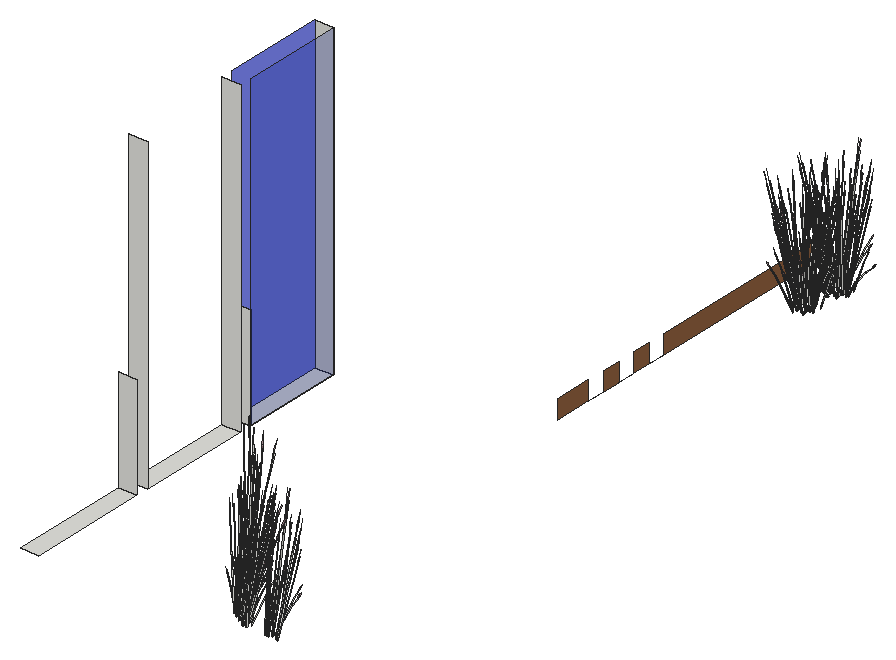
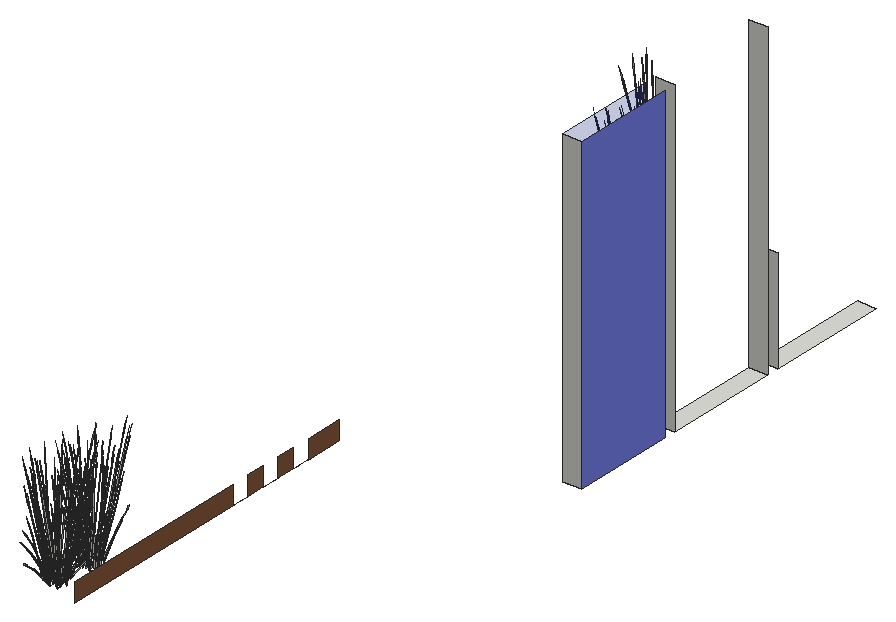
# SketchUp Ruby script. Lengths in inches.
U = 1.inch
M = Sketchup.active_model
def pt(a) = Geom::Point3d.new(a.map { |v| v * U })
def face(e, loops, mat)
  f = e.add_face(loops[0].map { |a| pt(a) })
  loops[1..].each { |l| e.add_face(l.map { |a| pt(a) }).erase! }
  f.material = f.back_material = mat if mat
  f
end
# faces: each face lists its corners as indices into pts; further lists are holes
def faces(e, pts, list, mat = nil) = list.each { |f| face(e, (f[0].is_a?(Array) ? f : [f]).map { |l| l.map { |i| pts[i] } }, mat) }
# xy, xz, yz: faces in a plane at the given z, y or x. An outline is a flat list of corners, or four numbers for a rectangle; further outlines are holes
def ring(l) = l.size == 4 ? [[l[0], l[1]], [l[2], l[1]], [l[2], l[3]], [l[0], l[3]]] : l.each_slice(2).to_a
def flat(e, list, mat, &to3) = list.each { |f| face(e, (f[0].is_a?(Array) ? f : [f]).map { |l| ring(l).map { |u, v| to3.(u, v) } }, mat) }
def xy(e, z, list, mat = nil) = flat(e, list, mat) { |x, y| [x, y, z] }
def xz(e, y, list, mat = nil) = flat(e, list, mat) { |x, z| [x, y, z] }
def yz(e, x, list, mat = nil) = flat(e, list, mat) { |y, z| [x, y, z] }
def lines(e, pts, list) = list.each { |a, b| e.add_line(pt(pts[a]), pt(pts[b])) }
# prism: a flat outline (further loops are holes) pulled along v
def prism(e, loops, v, mat = nil)
  f = face(e, loops, mat); d = Geom::Vector3d.new(v.map { |x| x * U })
  f.pushpull(f.normal.samedirection?(d) ? d.length : -d.length)
end
def box(e, o, s, mat = nil) = prism(e, [[o, [o[0] + s[0], o[1], o[2]], [o[0] + s[0], o[1] + s[1], o[2]], [o[0], o[1] + s[1], o[2]]]], [0, 0, s[2]], mat)
def at(x, y, z, deg = 0) = Geom::Transformation.translation(pt([x, y, z])) * Geom::Transformation.rotation(ORIGIN, Z_AXIS, deg.degrees)
def axes(o, x, y, z) = Geom::Transformation.new([*x, 0, *y, 0, *z, 0, *pt(o).to_a, 1])
def part(name) = M.definitions.add(name)
# library, detail: a bought-in or finely detailed component or shape, given as its bounding box
def library(name, o, s) = part(name).tap { |d| box(d.entities, o, s) }
def detail(e, o, s) = box(e.add_group.entities, o, s)
def put(e, d, t, mat = nil) = e.add_instance(d, t).tap { |i| i.material = mat if mat }
def group(e, t, mat = nil) = e.add_group.tap { |g| g.transformation = t; g.material = mat if mat }.entities
root = M.entities
M.materials.add("Glass_Basic_01").color = [23, 48, 186]
M.materials["Glass_Basic_01"].alpha = 0.25
M.materials.add("I03_Bluebell_Mist").color = [130, 140, 255]
M.materials.add("LightPink_Translucent").color = [144, 107, 117]
M.materials["LightPink_Translucent"].alpha = 0.75
M.materials.add("Wood_Veneer_15_1K").color = [142, 95, 62]
c1 = part("blade")
p = [[2.15,0.21,22],[0,0.17,0],[0.09,0.45,0],[2.18,0.31,22],[2.29,0.31,22],[0.38,0.45,0],
  [2.48,0.24,33],[2.49,0.24,33],[2.48,0.22,33]]
faces(c1.entities,p,[[0,1,2,3],[4,5,2,3],[6,3,4,7],[8,0,3,6]])
c2 = part("seeds")
p = [[0.3,-0.1,1.38],[-0.01,-0.03,1.59],[-0.01,-0.03,0.03],[0.14,-0.07,-0.07],[0.29,-0.03,3],[0.15,0.01,3.11]]
faces(c2.entities,p,[[0,1,2,3],[1,0,4,5]],"LightPink_Translucent")
c3 = part("blade with seeds")
put(c3.entities,c1,at(0,0,0))
put(c3.entities,c2,axes([2.4,0.25,30.99],[1.5799,-0.05474,1.17369],[-0.12525,1.92788,0.29478],[-0.07173,-0.02425,1.56792]))
xy(root,156.54,[[297,108,303,147],[297,151,303,188],[297,192,303,225]])
xz(root,147,[[297,156.54,303,189.54]])
xz(root,151,[[297,156.54,303,255.54]])
xz(root,188,[[297,156.54,303,255.54]])
xz(root,192,[[297,156.54,303,189.54]])
xz(root,225,[[297,156.54,303,255.54]])
yz(root,297,[[192,156.54,225,255.54]],"I03_Bluebell_Mist")
yz(root,303,[[192,156.54,225,255.54]],"Glass_Basic_01")
yz(root,360,[[243,156,255,162],[261,156,267,162],[273,156,279,162],[285,156,348,162]],"Wood_Veneer_15_1K")
p = [[360,242.96,156],[360,243,156],[360,255,156],[360,261,156],[360,267,156],[360,273,156],
  [360,279,156],[360,285,156]]
lines(root,p,[[0,1],[2,3],[4,5],[6,7]])
put(root,c3,axes([365.29,113.04,155.76],[-0.61202,-0.00483,-0.04678],[0,-0.67471,0.46946],[-0.01923,0.15359,1.48851]))
put(root,c3,axes([363.97,112.45,156.2],[0.55148,0.28805,-0.2735],[-0.26554,0.60796,-0.47002],[0.01733,0.14927,1.50125]))
put(root,c3,axes([360.12,114.69,156.3],[0.20408,-0.2736,1.07969],[0.08053,0.43313,0.79328],[-0.14748,0.07756,0.23781]))
put(root,c3,axes([365.03,114.18,157.95],[0.27863,0.37797,-0.33289],[-0.31815,0.35779,0.42977],[0.16164,0.05444,0.82232]))
put(root,c3,axes([365.17,113.13,155.6],[-0.34183,0.37665,-0.29119],[-0.34183,-0.37665,0.29119],[0,0.12132,1.30635]))
put(root,c3,axes([363.69,113.17,156.2],[0.05706,0.68884,-0.2735],[-0.59432,0.04165,-0.47002],[-0.10465,0.09176,1.50125]))
put(root,c3,axes([373.93,114.33,154.45],[-0.02466,0.45905,0.06044],[-0.37234,-0.01259,0.47584],[0.14263,0.04803,0.72558]))
put(root,c3,axes([364.89,114.33,158.14],[-0.02466,0.45905,0.06044],[-0.37234,-0.01259,0.47584],[0.14263,0.04803,0.72558]))
put(root,c3,axes([363.91,112.9,155.77],[-0.23759,0.54397,-0.42055],[-0.49367,-0.26179,0.2024],[0,0.12539,1.35025]))
put(root,c3,axes([360.89,113.51,157.95],[-0.42626,0.08628,-0.33289],[-0.11256,-0.4932,0.42977],[-0.12215,0.13247,0.82232]))
put(root,c3,axes([373.97,114.18,154.45],[-0.36108,0.39778,0.45122],[-0.31141,-0.42243,0.37205],[0.1694,0.07337,0.9337]))
put(root,c3,axes([364.93,114.18,158.15],[-0.36108,0.39778,0.45122],[-0.31141,-0.42243,0.37205],[0.1694,0.07337,0.9337]))
put(root,c3,axes([369.3125,114.62,155.31],[0.43212,0.16114,-0.06098],[-0.13292,0.49597,-0.27651],[-0.07068,0.0753,0.91203]))
put(root,c3,axes([360.27,114.62,159],[0.43212,0.16114,-0.06098],[-0.13292,0.49597,-0.27651],[-0.07068,0.0753,0.91203]))
put(root,c3,axes([372.82,114.64,154.75],[-0.07563,-0.48625,0.33289],[0.43235,-0.1284,-0.42977],[0.11613,0.13934,0.82232]))
put(root,c3,axes([363.78,114.64,158.44],[-0.07563,-0.48625,0.33289],[0.43235,-0.1284,-0.42977],[0.11613,0.13934,0.82232]))
put(root,c3,axes([363.92,114.46,155.89],[0.61306,0.19622,0.28911],[-0.15337,0.70136,-0.34302],[-0.10147,0.08778,1.54992]))
put(root,c3,axes([364.03,113.22,157.34],[-0.1819,-0.10401,1.61094],[0.37643,-0.43634,0.13026],[0.23461,0.19684,0.68866]))
put(root,c3,axes([364.07,111.85,157.9],[-0.42314,-0.31366,1.29986],[0.4468,-0.48836,0.56085],[0.13652,0.29431,1.25644]))
put(root,c3,axes([361.02,113.17,158.43],[0.45297,0.33287,-0.11431],[-0.26096,0.48206,-0.63445],[-0.12798,0.16757,0.96403]))
put(root,c3,axes([364.71,114.4,156.3],[-0.27572,-0.17358,1.07969],[0.35602,-0.17637,0.79328],[0.09603,0.1494,0.23781]))
put(root,c3,axes([363.74,114.9,158.43],[0.2918,-0.51673,-0.11431],[0.42258,0.29769,-0.63445],[0.14689,0.14599,0.96403]))
put(root,c3,axes([361.63,113.02,157.34],[0.12231,-0.18549,1.61094],[0.30882,0.50067,0.13026],[-0.21182,0.22801,0.68866]))
put(root,c3,axes([361.24,113.56,158.1],[0.1258,0.55122,-0.48033],[-0.4764,0.09643,-0.37205],[-0.13652,0.14806,0.91906]))
put(root,c3,axes([370.85,114.2,154.75],[0.33133,-0.31784,0.33289],[0.31365,0.36292,-0.42977],[-0.04772,0.1844,0.82232]))
put(root,c3,axes([361.81,114.2,158.44],[0.33133,-0.31784,0.33289],[0.31365,0.36292,-0.42977],[-0.04772,0.1844,0.82232]))
put(root,c3,axes([364.3,114.84,155.93],[0.30616,0.60492,0],[-0.51222,0.33735,-0.48511],[-0.11666,0.07683,1.53889]))
put(root,c3,axes([372.4,115.32,154.43],[0.00145,-0.07309,1.6674],[0.41965,-0.32245,-0.15755],[0.14577,0.11509,0.29507]))
put(root,c3,axes([363.36,115.32,158.12],[0.00145,-0.07309,1.6674],[0.41965,-0.32245,-0.15755],[0.14577,0.11509,0.29507]))
put(root,c3,axes([364.78,115.05,155.1],[0.03568,-0.08715,1.65762],[0.44916,-0.25668,-0.25323],[0.13617,0.13285,0.28235]))
put(root,c3,axes([364.04,112.45,156.37],[-0.01338,-0.56839,1.32796],[0.60542,0.14734,0.56227],[-0.14319,0.31102,1.25349]))
put(root,c3,axes([370.55,114.49,154.45],[-0.40242,-0.02813,0.06044],[0.01103,-0.42474,0.47584],[-0.04211,0.1627,0.72558]))
put(root,c3,axes([361.51,114.49,158.14],[-0.40242,-0.02813,0.06044],[0.01103,-0.42474,0.47584],[-0.04211,0.1627,0.72558]))
put(root,c3,axes([360.66,114.97,155.1],[0.06569,0.06031,1.65762],[0.11138,0.55882,-0.25323],[-0.14558,0.11917,0.28235]))
put(root,c3,axes([370.68,114.53,154.45],[-0.3487,-0.41189,0.45122],[0.37031,-0.35523,0.37205],[-0.06432,0.19325,0.9337]))
put(root,c3,axes([361.64,114.53,158.15],[-0.3487,-0.41189,0.45122],[0.37031,-0.35523,0.37205],[-0.06432,0.19325,0.9337]))
put(root,c3,axes([364.08,114.64,158.1],[0.48321,-0.1435,-0.48033],[0.08453,0.54345,-0.37205],[0.12979,0.15574,0.91906]))
put(root,c3,axes([371.78,114.72,154.75],[0.14763,-0.46424,0.33289],[0.4307,0.1354,-0.42977],[0.03949,0.18691,0.82232]))
put(root,c3,axes([362.74,114.72,158.44],[0.14763,-0.46424,0.33289],[0.4307,0.1354,-0.42977],[0.03949,0.18691,0.82232]))
put(root,c3,axes([364.75,115.19,156.2],[-0.31402,-0.01893,0.98757],[0.20738,-0.40212,0.54525],[0.12405,0.14286,0.77466]))
put(root,c3,axes([372.89,115.08,154.45],[-0.22256,0.38349,0.06044],[-0.31694,-0.22327,0.47584],[0.10247,0.12295,0.72558]))
put(root,c3,axes([363.85,115.08,158.14],[-0.22256,0.38349,0.06044],[-0.31694,-0.22327,0.47584],[0.10247,0.12295,0.72558]))
put(root,c3,axes([372.36,116.38,155.31],[0.3384,-0.34633,-0.06098],[0.31006,0.3793,-0.27651],[0.02183,0.10747,0.91203]))
put(root,c3,axes([363.32,116.38,159],[0.3384,-0.34633,-0.06098],[0.31006,0.3793,-0.27651],[0.02183,0.10747,0.91203]))
put(root,c3,axes([372.98,114.98,154.45],[-0.48705,0.13854,0.45122],[-0.08453,-0.54345,0.37205],[0.11455,0.16017,0.9337]))
put(root,c3,axes([363.94,114.98,158.15],[-0.48705,0.13854,0.45122],[-0.08453,-0.54345,0.37205],[0.11455,0.16017,0.9337]))
put(root,c3,axes([361.54,113.48,157.34],[0.09118,-0.2075,1.61094],[0.3825,0.42941,0.13026],[-0.17255,0.26763,0.68866]))
put(root,c3,axes([363.73,114.22,156.13],[0.00864,-0.20012,1.34422],[0.41296,-0.22353,-0.28909],[0.12748,0.23952,0.57472]))
put(root,c3,axes([371.65,115.14,154.45],[-0.36083,0.20517,0.06044],[-0.17661,-0.37413,0.47584],[0.03485,0.16492,0.72558]))
put(root,c3,axes([362.61,115.14,158.14],[-0.36083,0.20517,0.06044],[-0.17661,-0.37413,0.47584],[0.03485,0.16492,0.72558]))
put(root,c3,axes([361.64,114.65,157.95],[-0.33133,0.31784,-0.33289],[-0.31365,-0.36292,0.42977],[-0.04772,0.1844,0.82232]))
put(root,c3,axes([369.54,114.55,154.43],[-0.01217,0.11946,1.64448],[0.34544,0.41559,-0.26007],[-0.09043,0.19653,0.13189]))
put(root,c3,axes([360.5,114.55,158.13],[-0.01217,0.11946,1.64448],[0.34544,0.41559,-0.26007],[-0.09043,0.19653,0.13189]))
put(root,c3,axes([370.64,114.29,155.07],[0.53819,0.02991,-0.12688],[-0.01471,0.56632,-0.70424],[-0.03738,0.21811,1.07008]))
put(root,c3,axes([361.6,114.29,158.77],[0.53819,0.02991,-0.12688],[-0.01471,0.56632,-0.70424],[-0.03738,0.21811,1.07008]))
put(root,c3,axes([362.6,114.92,158.43],[0.47919,-0.28106,-0.11431],[0.23549,0.49884,-0.63445],[0.06322,0.21021,0.96403]))
put(root,c3,axes([371.78,115.1,154.76],[-0.48252,-0.15782,0.50086],[0.165,-0.51886,0.41298],[0.029,0.20404,1.03641]))
put(root,c3,axes([362.74,115.1,158.46],[-0.48252,-0.15782,0.50086],[0.165,-0.51886,0.41298],[0.029,0.20404,1.03641]))
put(root,c3,axes([361.85,115.88,156.3],[-0.01267,-0.35895,1.07969],[0.31667,0.25602,0.79328],[-0.06228,0.17109,0.23781]))
put(root,c3,axes([362.6875,115.03,155.1],[0.07925,-0.03285,1.65762],[0.47671,0.18081,-0.25323],[0.01394,0.20378,0.28235]))
put(root,c3,axes([361.97,114.5,158.4],[0.35055,0.40562,-0.53317],[-0.37031,0.35523,-0.41298],[-0.05334,0.20609,1.02016]))
put(root,c3,axes([361.59,115.11,156.35],[0.44486,-0.1069,0.06117],[0.10227,0.43069,-0.81126],[-0.0282,0.21802,0.72719]))
put(root,c3,axes([363.01,114.89,158.1],[0.48137,0.15133,-0.48033],[-0.165,0.51886,-0.37205],[0.04414,0.2089,0.91906]))
put(root,c3,axes([363.28,113.82,157.34],[-0.11194,-0.19382,1.61094],[0.51725,-0.16318,0.13026],[0.1169,0.30428,0.68866]))
put(root,c3,axes([362.79,115.21,157.95],[-0.14763,0.46424,-0.33289],[-0.4307,-0.1354,0.42977],[0.03949,0.18691,0.82232]))
put(root,c3,axes([361.86,114.3125,158.71],[-0.01274,0.55841,-0.74129],[-0.53656,-0.0375,0.08946],[-0.05662,0.23657,1.04862]))
put(root,c3,axes([369.5,115.78,154.43],[0.05555,-0.03645,1.6674],[0.45917,0.24243,-0.15755],[-0.01079,0.20185,0.29507]))
put(root,c3,axes([360.46,115.78,158.12],[0.05555,-0.03645,1.6674],[0.45917,0.24243,-0.15755],[-0.01079,0.20185,0.29507]))
put(root,c3,axes([362.37,113.92,157.34],[-0.01199,-0.2317,1.61094],[0.51947,0.15371,0.13026],[-0.03213,0.3302,0.68866]))
put(root,c3,axes([362.84,114.79,158.38],[0.23372,0.49086,-0.66783],[-0.48111,0.27356,0.08059],[0.05465,0.23717,0.9447]))
put(root,c3,axes([361.48,115.57,156.13],[0.15453,-0.09523,1.34422],[0.38153,0.28715,-0.28909],[-0.11356,0.24846,0.57472]))
put(root,c3,axes([371.53,116.03,154.43],[0.06207,0.09721,1.64448],[0.50093,0.03819,-0.26007],[0.05037,0.21439,0.13189]))
put(root,c3,axes([362.49,116.03,158.13],[0.06207,0.09721,1.64448],[0.50093,0.03819,-0.26007],[0.05037,0.21439,0.13189]))
put(root,c3,axes([361.68,115.1,156.86],[0.01076,-0.31164,1.45085],[0.48391,0.16461,0.20049],[-0.04193,0.33214,0.68509]))
put(root,c3,axes([372.83,324.64,154.43],[-0.04973,0.04611,1.6674],[-0.48725,-0.15557,-0.15755],[-0.01764,-0.20123,0.29507]))
put(root,c3,axes([370.18,323.75,154.43],[-0.00914,0.07236,1.6674],[-0.45057,0.26261,-0.15755],[-0.13259,-0.13424,0.29507]))
put(root,c3,axes([370.08,325.04,154.79],[0.5455,-0.15516,0.50537],[0.09467,0.60867,0.4167],[-0.12829,-0.17939,1.04574]))
put(root,c3,axes([371.31,325.15,154.45],[0.48252,0.15782,0.45122],[-0.165,0.51886,0.37205],[-0.029,-0.20404,0.9337]))
put(root,c3,axes([371.4375,325.11,154.45],[0.36083,-0.20517,0.06044],[0.17661,0.37413,0.47584],[-0.03485,-0.16492,0.72558]))
put(root,c3,axes([370.2,325.17,154.45],[0.22256,-0.38349,0.06044],[0.31694,0.22327,0.47584],[-0.10247,-0.12295,0.72558]))
put(root,c3,axes([371.3,325.53,154.75],[-0.14763,0.46424,0.33289],[-0.4307,-0.1354,-0.42977],[-0.03949,-0.18691,0.82232]))
put(root,c3,axes([372.41,325.73,154.45],[0.3487,0.41189,0.45122],[-0.37031,0.35523,0.37205],[0.06432,-0.19325,0.9337]))
put(root,c3,axes([370.3,325.13,155.1],[-0.32682,0.57873,-0.12802],[-0.47329,-0.33342,-0.71058],[-0.16452,-0.16351,1.07972]))
put(root,c3,axes([372.53,325.77,154.45],[0.40242,0.02813,0.06044],[-0.01103,0.42474,0.47584],[0.04211,-0.1627,0.72558]))
put(root,c3,axes([372.23,326.06,154.75],[-0.33133,0.31784,0.33289],[-0.31365,-0.36292,-0.42977],[0.04772,-0.1844,0.82232]))
put(root,c3,axes([370.27,325.61,154.75],[0.07563,0.48625,0.33289],[-0.43235,0.1284,-0.42977],[-0.11613,-0.13934,0.82232]))
put(root,c3,axes([368.97,325.93,154.79],[0.4044,-0.44551,0.50537],[0.34877,0.47312,0.4167],[-0.18973,-0.08218,1.04574]))
put(root,c3,axes([374.15,326.94,154.43],[-0.06396,-0.00458,1.6674],[-0.2656,-0.49127,-0.15755],[0.10666,-0.16153,0.29507]))
put(root,c3,axes([369.16,325.92,154.45],[0.02466,-0.45905,0.06044],[0.37234,0.01259,0.47584],[-0.14263,-0.04803,0.72558]))
put(root,c3,axes([372.81,327.04,154.75],[-0.42626,0.08628,0.33289],[-0.11256,-0.4932,-0.42977],[0.12215,-0.13247,0.82232]))
put(root,c3,axes([373.2,326.96,154.45],[0.33617,0.25389,0.06044],[-0.19572,0.36154,0.47584],[0.10778,-0.11689,0.72558]))
put(root,c3,axes([373.1,326.85,154.45],[0.12145,0.5556,0.45122],[-0.4764,0.09643,0.37205],[0.14041,-0.13067,0.9337]))
put(root,c3,axes([368.64,325.33,154.43],[0.0363,0.06025,1.6674],[-0.17501,0.54156,-0.15755],[-0.17724,0.00392,0.29507]))
put(root,c3,axes([369.41,326.27,154.75],[0.27863,0.37797,0.33289],[-0.31815,0.35779,-0.42977],[-0.16164,-0.05444,0.82232]))
put(root,c3,axes([372.875,328.22,154.75],[-0.40696,-0.16841,0.33289],[0.1187,-0.49132,-0.42977],[0.16385,-0.04505,0.82232]))
put(root,c3,axes([368.62,327.32,154.45],[0.13835,-0.55043,0.45122],[0.45484,0.18822,0.37205],[-0.17887,0.03308,0.9337]))
put(root,c3,axes([368.58,327.17,154.45],[-0.17985,-0.41162,0.06044],[0.32797,-0.20147,0.47584],[-0.14457,0.03975,0.72558]))
put(root,c3,axes([373.25,328.37,154.45],[0.17985,0.41162,0.06044],[-0.32797,0.20147,0.47584],[0.14457,-0.03975,0.72558]))
put(root,c3,axes([373.21,328.23,154.45],[-0.13835,0.55043,0.45122],[-0.45484,-0.18822,0.37205],[0.17887,-0.03308,0.9337]))
put(root,c3,axes([368.95,327.33,154.75],[0.40696,0.16841,0.33289],[-0.1187,0.49132,-0.42977],[-0.16385,0.04505,0.82232]))
put(root,c3,axes([374.03,330.01,154.43],[-0.04428,-0.05285,1.6674],[0.09686,-0.56651,-0.15755],[0.17442,-0.03619,0.29507]))
put(root,c3,axes([372.42,329.28,154.75],[-0.27863,-0.37797,0.33289],[0.31815,-0.35779,-0.42977],[0.16164,0.05444,0.82232]))
put(root,c3,axes([368.73,328.69,154.45],[-0.12145,-0.5556,0.45122],[0.4764,-0.09643,0.37205],[-0.14041,0.13067,0.9337]))
put(root,c3,axes([368.63,328.58,154.45],[-0.33617,-0.25389,0.06044],[0.19572,-0.36154,0.47584],[-0.10778,0.11689,0.72558]))
put(root,c3,axes([369.02,328.51,154.75],[0.42626,-0.08628,0.33289],[0.11256,0.4932,-0.42977],[-0.12215,0.13247,0.82232]))
put(root,c3,axes([367.375,328.29,154.43],[0.06249,0.01619,1.6674],[0.19333,0.53339,-0.15755],[-0.12793,0.14,0.29507]))
put(root,c3,axes([372.67,329.62,154.45],[-0.02466,0.45905,0.06044],[-0.37234,-0.01259,0.47584],[0.14263,0.04803,0.72558]))
put(root,c3,axes([372.71,329.47,154.45],[-0.36108,0.39778,0.45122],[-0.31141,-0.42243,0.37205],[0.1694,0.07337,0.9337]))
put(root,c3,axes([368.05,329.91,155.31],[0.43212,0.16114,-0.06098],[-0.13292,0.49597,-0.27651],[-0.07068,0.0753,0.91203]))
put(root,c3,axes([371.56,329.93,154.75],[-0.07563,-0.48625,0.33289],[0.43235,-0.1284,-0.42977],[0.11613,0.13934,0.82232]))
put(root,c3,axes([371.95,335.66,154.43],[-0.0749,-0.08464,1.64448],[-0.49984,0.05366,-0.26007],[-0.07977,-0.20245,0.13189]))
put(root,c3,axes([369.59,329.49,154.75],[0.33133,-0.31784,0.33289],[0.31365,0.36292,-0.42977],[-0.04772,0.1844,0.82232]))
put(root,c3,axes([371.14,330.62,154.43],[0.00145,-0.07309,1.6674],[0.41965,-0.32245,-0.15755],[0.14577,0.11509,0.29507]))
put(root,c3,axes([369.29,329.78,154.45],[-0.40242,-0.02813,0.06044],[0.01103,-0.42474,0.47584],[-0.04211,0.1627,0.72558]))
put(root,c3,axes([374.19,336.7,154.43],[-0.00473,-0.12015,1.64448],[-0.39924,-0.34724,-0.26007],[0.06173,-0.21049,0.13189]))
put(root,c3,axes([369.42,329.82,154.45],[-0.3487,-0.41189,0.45122],[0.37031,-0.35523,0.37205],[-0.06432,0.19325,0.9337]))
put(root,c3,axes([374.09,336.27,154.43],[-0.04973,0.04611,1.6674],[-0.48725,-0.15557,-0.15755],[-0.01764,-0.20123,0.29507]))
put(root,c3,axes([370.52,330.01,154.75],[0.14763,-0.46424,0.33289],[0.4307,0.1354,-0.42977],[0.03949,0.18691,0.82232]))
put(root,c3,axes([371.625,330.375,154.45],[-0.22256,0.38349,0.06044],[-0.31694,-0.22327,0.47584],[0.10247,0.12295,0.72558]))
put(root,c3,axes([371.4375,335.38,154.43],[-0.00914,0.07236,1.6674],[-0.45057,0.26261,-0.15755],[-0.13259,-0.13424,0.29507]))
put(root,c3,axes([371.1,331.67,155.31],[0.3384,-0.34633,-0.06098],[0.31006,0.3793,-0.27651],[0.02183,0.10747,0.91203]))
put(root,c3,axes([371.72,330.27,154.45],[-0.48705,0.13854,0.45122],[-0.08453,-0.54345,0.37205],[0.11455,0.16017,0.9337]))
put(root,c3,axes([371.34,336.67,154.79],[0.5455,-0.15516,0.50537],[0.09467,0.60867,0.4167],[-0.12829,-0.17939,1.04574]))
put(root,c3,axes([372.57,336.78,154.45],[0.48252,0.15782,0.45122],[-0.165,0.51886,0.37205],[-0.029,-0.20404,0.9337]))
put(root,c3,axes([372.7,336.74,154.45],[0.36083,-0.20517,0.06044],[0.17661,0.37413,0.47584],[-0.03485,-0.16492,0.72558]))
put(root,c3,axes([370.39,330.43,154.45],[-0.36083,0.20517,0.06044],[-0.17661,-0.37413,0.47584],[0.03485,0.16492,0.72558]))
put(root,c3,axes([369.38,329.58,155.07],[0.53819,0.02991,-0.12688],[-0.01471,0.56632,-0.70424],[-0.03738,0.21811,1.07008]))
put(root,c3,axes([370.52,330.39,154.76],[-0.48252,-0.15782,0.50086],[0.165,-0.51886,0.41298],[0.029,0.20404,1.03641]))
put(root,c3,axes([371.46,336.8,154.45],[0.22256,-0.38349,0.06044],[0.31694,0.22327,0.47584],[-0.10247,-0.12295,0.72558]))
put(root,c3,axes([372.56,337.16,154.75],[-0.14763,0.46424,0.33289],[-0.4307,-0.1354,-0.42977],[-0.03949,-0.18691,0.82232]))
put(root,c3,axes([373.67,337.36,154.45],[0.3487,0.41189,0.45122],[-0.37031,0.35523,0.37205],[0.06432,-0.19325,0.9337]))
put(root,c3,axes([371.5625,336.76,155.1],[-0.32682,0.57873,-0.12802],[-0.47329,-0.33342,-0.71058],[-0.16452,-0.16351,1.07972]))
put(root,c3,axes([373.79,337.4,154.45],[0.40242,0.02813,0.06044],[-0.01103,0.42474,0.47584],[0.04211,-0.1627,0.72558]))
put(root,c3,axes([368.24,331.07,154.43],[0.05555,-0.03645,1.6674],[0.45917,0.24243,-0.15755],[-0.01079,0.20185,0.29507]))
put(root,c3,axes([373.49,337.68,154.75],[-0.33133,0.31784,0.33289],[-0.31365,-0.36292,-0.42977],[0.04772,-0.1844,0.82232]))
put(root,c3,axes([370.31,336.59,154.43],[-0.10536,-0.00426,1.64448],[-0.33544,0.42612,-0.26007],[-0.17898,-0.08707,0.13189]))
put(root,c3,axes([371.53,337.24,154.75],[0.07563,0.48625,0.33289],[-0.43235,0.1284,-0.42977],[-0.11613,-0.13934,0.82232]))
put(root,c3,axes([370.23,337.56,154.79],[0.4044,-0.44551,0.50537],[0.34877,0.47312,0.4167],[-0.18973,-0.08218,1.04574]))
put(root,c3,axes([375.41,338.57,154.43],[-0.06396,-0.00458,1.6674],[-0.2656,-0.49127,-0.15755],[0.10666,-0.16153,0.29507]))
put(root,c3,axes([370.42,337.55,154.45],[0.02466,-0.45905,0.06044],[0.37234,0.01259,0.47584],[-0.14263,-0.04803,0.72558]))
put(root,c3,axes([374.07,338.67,154.75],[-0.42626,0.08628,0.33289],[-0.11256,-0.4932,-0.42977],[0.12215,-0.13247,0.82232]))
put(root,c3,axes([374.46,338.59,154.45],[0.33617,0.25389,0.06044],[-0.19572,0.36154,0.47584],[0.10778,-0.11689,0.72558]))
put(root,c3,axes([374.36,338.48,154.45],[0.12145,0.5556,0.45122],[-0.4764,0.09643,0.37205],[0.14041,-0.13067,0.9337]))
put(root,c3,axes([375.65,339.15,154.43],[0.06795,-0.09195,1.64448],[-0.08698,-0.56405,-0.26007],[0.1705,-0.10694,0.13189]))
put(root,c3,axes([369.9,336.95,154.43],[0.0363,0.06025,1.6674],[-0.17501,0.54156,-0.15755],[-0.17724,0.00392,0.29507]))
put(root,c3,axes([370.67,337.9,154.75],[0.27863,0.37797,0.33289],[-0.31815,0.35779,-0.42977],[-0.16164,-0.05444,0.82232]))
put(root,c3,axes([374.14,339.85,154.75],[-0.40696,-0.16841,0.33289],[0.1187,-0.49132,-0.42977],[0.16385,-0.04505,0.82232]))
put(root,c3,axes([369.875,338.95,154.45],[0.13835,-0.55043,0.45122],[0.45484,0.18822,0.37205],[-0.17887,0.03308,0.9337]))
put(root,c3,axes([369.84,338.8,154.45],[-0.17985,-0.41162,0.06044],[0.32797,-0.20147,0.47584],[-0.14457,0.03975,0.72558]))
put(root,c3,axes([374.51,340,154.45],[0.17985,0.41162,0.06044],[-0.32797,0.20147,0.47584],[0.14457,-0.03975,0.72558]))
put(root,c3,axes([374.47,339.85,154.45],[-0.13835,0.55043,0.45122],[-0.45484,-0.18822,0.37205],[0.17887,-0.03308,0.9337]))
put(root,c3,axes([370.21,338.96,154.75],[0.40696,0.16841,0.33289],[-0.1187,0.49132,-0.42977],[-0.16385,0.04505,0.82232]))
put(root,c3,axes([375.29,341.64,154.43],[-0.04428,-0.05285,1.6674],[0.09686,-0.56651,-0.15755],[0.17442,-0.03619,0.29507]))
put(root,c3,axes([369.53,339.34,154.43],[-0.07997,0.07838,1.64448],[0.0068,0.57266,-0.26007],[-0.1833,0.07447,0.13189]))
put(root,c3,axes([373.68,340.91,154.75],[-0.27863,-0.37797,0.33289],[0.31815,-0.35779,-0.42977],[0.16164,0.05444,0.82232]))
put(root,c3,axes([374.1875,340.78,154.43],[0.10505,-0.01021,1.64448],[0.28813,-0.469,-0.26007],[0.18685,0.06191,0.13189]))
put(root,c3,axes([369.99,340.32,154.45],[-0.12145,-0.5556,0.45122],[0.4764,-0.09643,0.37205],[-0.14041,0.13067,0.9337]))
put(root,c3,axes([369.89,340.21,154.45],[-0.33617,-0.25389,0.06044],[0.19572,-0.36154,0.47584],[-0.10778,0.11689,0.72558]))
put(root,c3,axes([370.28,340.13,154.75],[0.42626,-0.08628,0.33289],[0.11256,0.4932,-0.42977],[-0.12215,0.13247,0.82232]))
put(root,c3,axes([368.64,339.92,154.43],[0.06249,0.01619,1.6674],[0.19333,0.53339,-0.15755],[-0.12793,0.14,0.29507]))
put(root,c3,axes([373.93,341.25,154.45],[-0.02466,0.45905,0.06044],[-0.37234,-0.01259,0.47584],[0.14263,0.04803,0.72558]))
put(root,c3,axes([373.97,341.1,154.45],[-0.36108,0.39778,0.45122],[-0.31141,-0.42243,0.37205],[0.1694,0.07337,0.9337]))
put(root,c3,axes([369.3125,341.54,155.31],[0.43212,0.16114,-0.06098],[-0.13292,0.49597,-0.27651],[-0.07068,0.0753,0.91203]))
put(root,c3,axes([372.82,341.5625,154.75],[-0.07563,-0.48625,0.33289],[0.43235,-0.1284,-0.42977],[0.11613,0.13934,0.82232]))
put(root,c3,axes([370.85,341.12,154.75],[0.33133,-0.31784,0.33289],[0.31365,0.36292,-0.42977],[-0.04772,0.1844,0.82232]))
put(root,c3,axes([372.4,342.24,154.43],[0.00145,-0.07309,1.6674],[0.41965,-0.32245,-0.15755],[0.14577,0.11509,0.29507]))
put(root,c3,axes([370.55,341.41,154.45],[-0.40242,-0.02813,0.06044],[0.01103,-0.42474,0.47584],[-0.04211,0.1627,0.72558]))
put(root,c3,axes([370.68,341.44,154.45],[-0.3487,-0.41189,0.45122],[0.37031,-0.35523,0.37205],[-0.06432,0.19325,0.9337]))
put(root,c3,axes([371.78,341.64,154.75],[0.14763,-0.46424,0.33289],[0.4307,0.1354,-0.42977],[0.03949,0.18691,0.82232]))
put(root,c3,axes([372.89,342,154.45],[-0.22256,0.38349,0.06044],[-0.31694,-0.22327,0.47584],[0.10247,0.12295,0.72558]))
put(root,c3,axes([372.36,343.3,155.31],[0.3384,-0.34633,-0.06098],[0.31006,0.3793,-0.27651],[0.02183,0.10747,0.91203]))
put(root,c3,axes([372.98,341.9,154.45],[-0.48705,0.13854,0.45122],[-0.08453,-0.54345,0.37205],[0.11455,0.16017,0.9337]))
put(root,c3,axes([371.65,342.0625,154.45],[-0.36083,0.20517,0.06044],[-0.17661,-0.37413,0.47584],[0.03485,0.16492,0.72558]))
put(root,c3,axes([369.54,341.47,154.43],[-0.01217,0.11946,1.64448],[0.34544,0.41559,-0.26007],[-0.09043,0.19653,0.13189]))
put(root,c3,axes([370.64,341.2,155.07],[0.53819,0.02991,-0.12688],[-0.01471,0.56632,-0.70424],[-0.03738,0.21811,1.07008]))
put(root,c3,axes([371.78,342.02,154.76],[-0.48252,-0.15782,0.50086],[0.165,-0.51886,0.41298],[0.029,0.20404,1.03641]))
put(root,c3,axes([369.5,342.7,154.43],[0.05555,-0.03645,1.6674],[0.45917,0.24243,-0.15755],[-0.01079,0.20185,0.29507]))
put(root,c3,axes([371.53,342.95,154.43],[0.06207,0.09721,1.64448],[0.50093,0.03819,-0.26007],[0.05037,0.21439,0.13189]))
